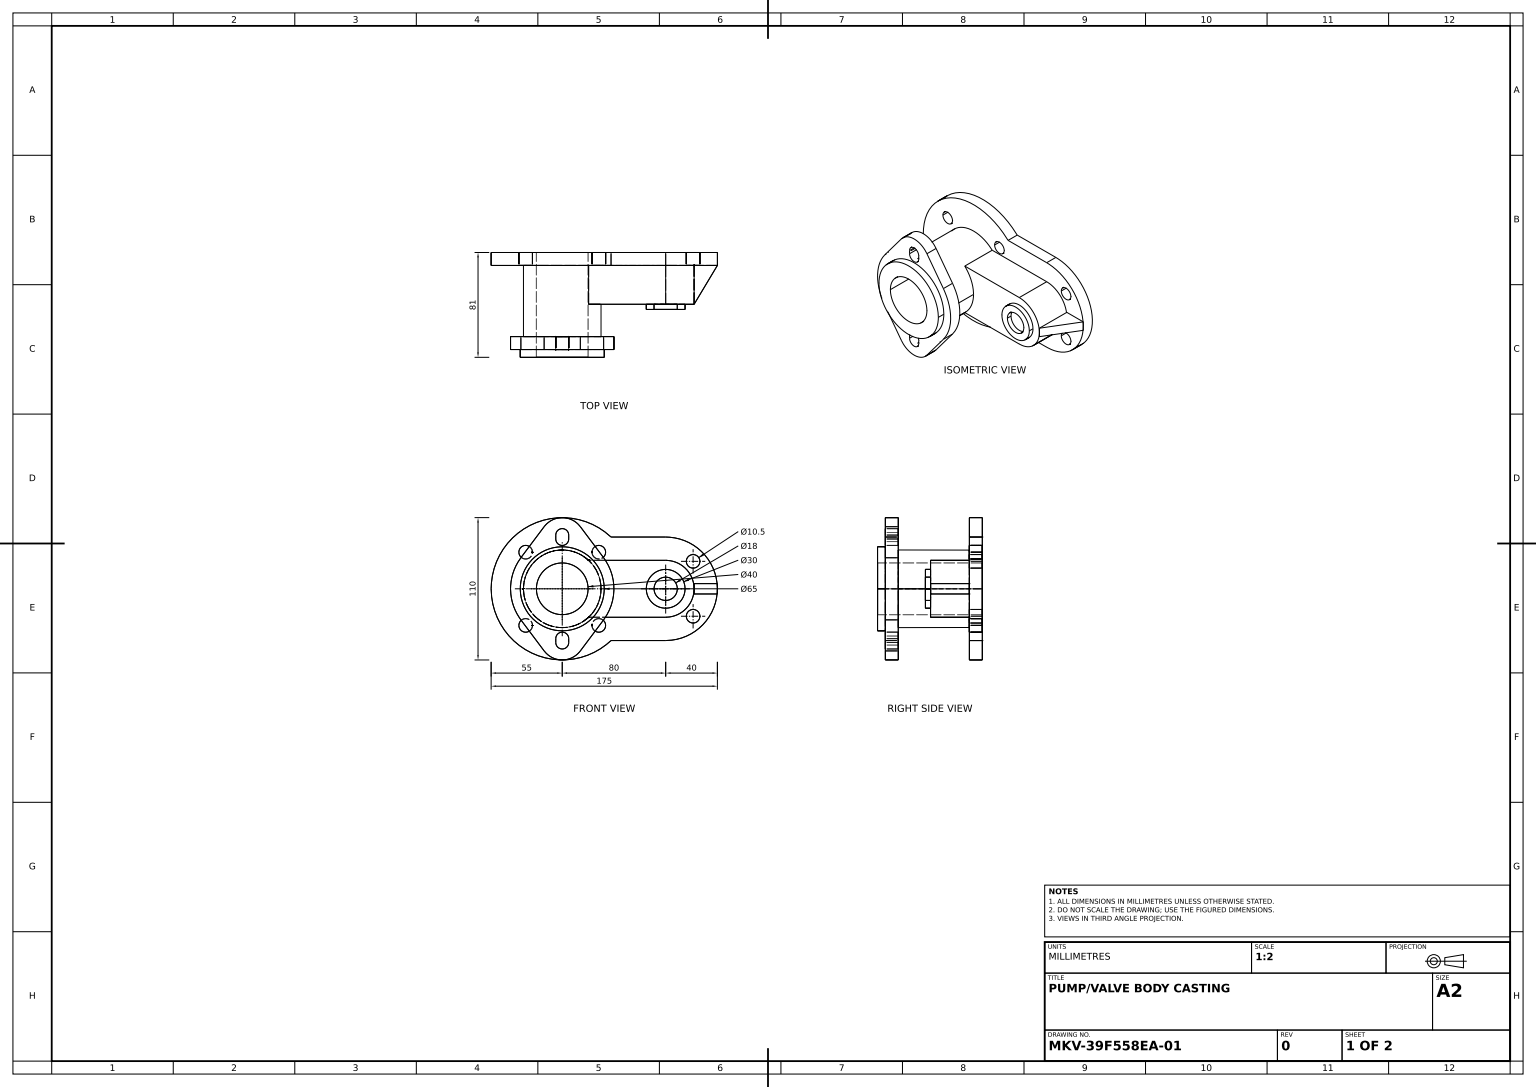
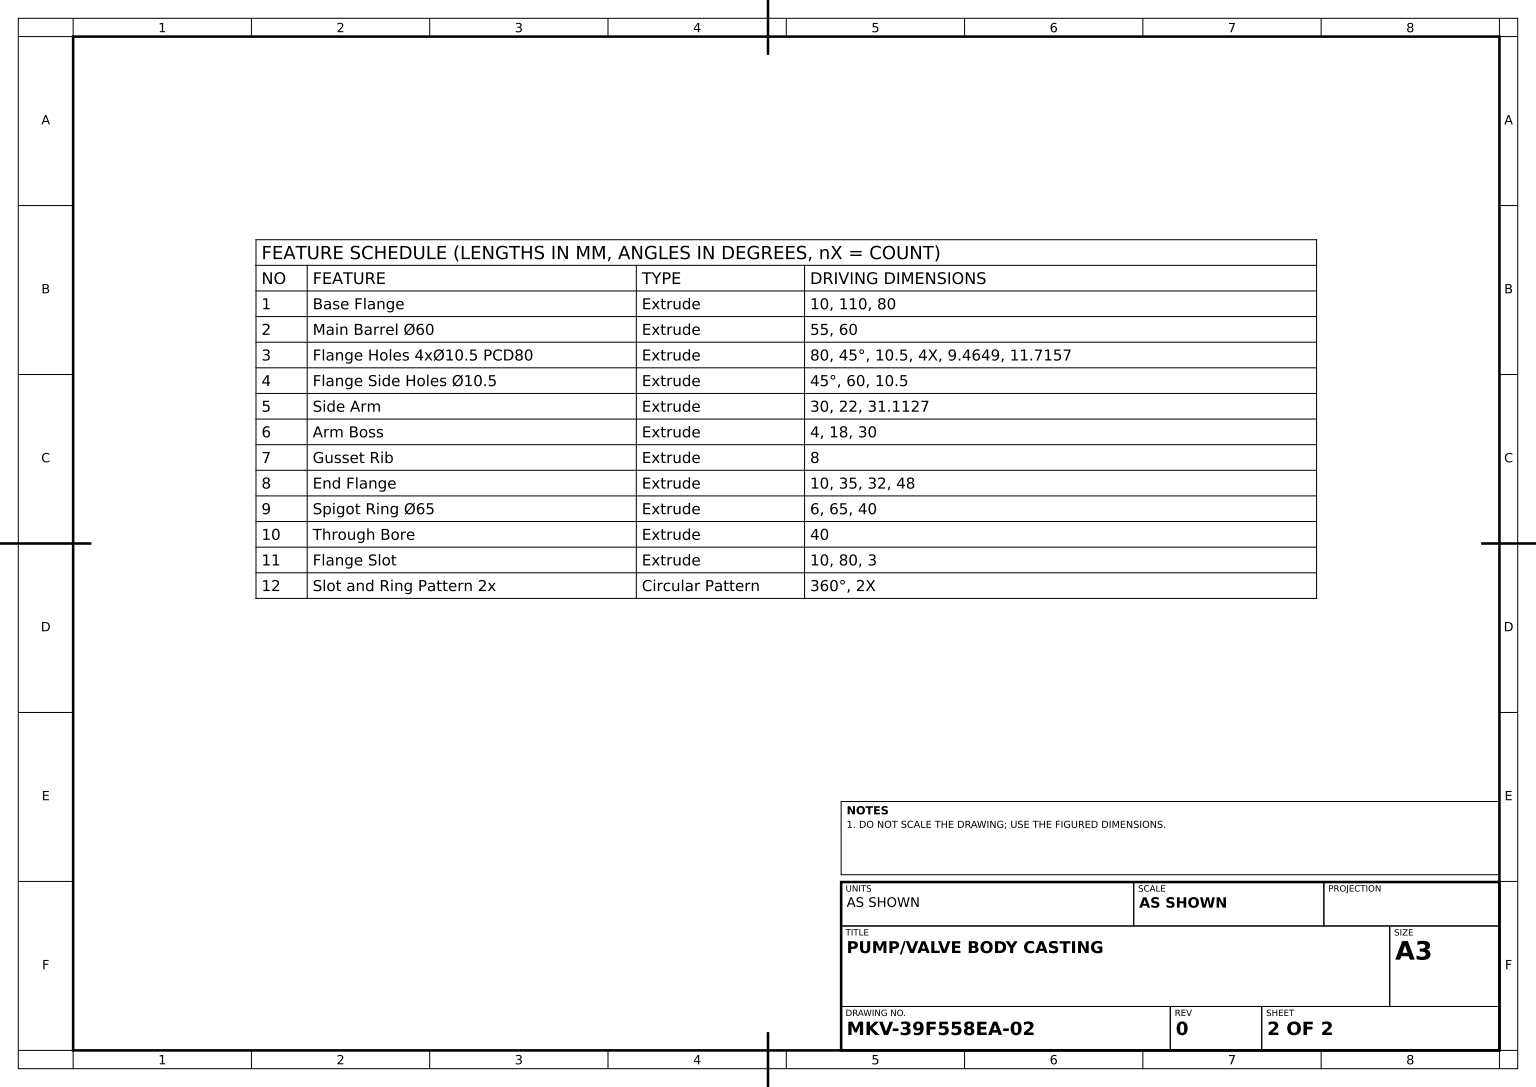
solid
v1 (102,4,40)
v2 (102,-4,40)
e1 v1 v2 LINE
v3 (102,4,10)
e2 v3 v1 LINE
v4 (102,-4,10)
e3 v3 v4 LINE
e4 v4 v2 LINE
face PLANE(AX(P(102,4,40),D(1,0,0),D(0,0,-1))) rev [-e1 -e2 e3 e4]
v5 (120,-4,10)
e5 v5 v4 LINE
v6 (120,4,10)
e6 v6 v3 LINE
e7 v6 v5 LINE
face PLANE(AX(P(102,4,10),D(0,0,1),D(1,0,0))) rev [e5 -e3 -e6 e7]
e8 v1 v6 LINE
face PLANE(AX(P(0,4,0),D(0,-1,0),D(0,0,-1))) rev [e6 e2 e8]
e9 v2 v5 LINE
face PLANE(AX(P(0,-4,0),D(0,-1,0),D(0,0,-1))) [-e4 -e5 -e9]
face PLANE(AX(P(102,4,40),D(-0.857492926,0,-0.514495755),D(-0.514495755,0,0.857492926))) rev [-e8 e1 e9 -e7]
solid
v7 (-5,41.5,65)
v8 (-5,41.5,75)
e10 v7 v8 LINE
v9 (5,41.5,65)
e11 v9 v7 CIRCLE(AX(P(0,41.5,65),D(0,0,1),D(1,0,0)),5)
v10 (5,41.5,75)
e12 v9 v10 LINE
e13 v10 v8 CIRCLE(AX(P(0,41.5,75),D(0,0,1),D(1,0,0)),5)
face CYL(AX(P(0,41.5,65),D(0,0,1),D(1,0,0)),5) rev [-e10 -e11 e12 e13]
v11 (80,-40,10)
v12 (80,-40,0)
e14 v11 v12 LINE
v13 (37.749172,-40,10)
e15 v13 v11 LINE
v14 (37.749172,-40,0)
e16 v13 v14 LINE
e17 v14 v12 LINE
face PLANE(AX(P(80,-40,10),D(0,1,0),D(0,0,1))) rev [-e14 -e15 e16 e17]
v15 (30,0,65)
v16 (-30,0,65)
e18 v15 v16 CIRCLE(AX(P(0,0,65),D(0,0,1),D(1,0,0)),30)
v17 (30,0,40)
e19 v15 v17 LINE
v18 (20.396078,22,40)
e20 v17 v18 CIRCLE(AX(P(0,0,40),D(0,0,1),D(1,0,0)),30)
v19 (20.396078,22,10)
e21 v18 v19 LINE
v20 (-30,0,10)
e22 v19 v20 CIRCLE(AX(P(0,0,10),D(0,0,1),D(1,0,0)),30)
e23 v16 v20 LINE
face CYL(AX(P(0,0,65),D(0,0,-1),D(-1,0,0)),30) [-e18 e19 e20 e21 e22 -e23]
v21 (-23.034271,-28.284271,10)
v22 (-33.534271,-28.284271,10)
e24 v21 v22 CIRCLE(AX(P(-28.284271,-28.284271,10),D(0,0,1),D(1,0,0)),5.25)
v23 (-33.534271,-28.284271,0)
e25 v23 v22 LINE
v24 (-23.034271,-28.284271,0)
e26 v24 v23 CIRCLE(AX(P(-28.284271,-28.284271,0),D(0,0,1),D(1,0,0)),5.25)
e27 v24 v21 LINE
face CYL(AX(P(-28.284271,-28.284271,0),D(0,0,1),D(1,0,0)),5.25) rev [e24 -e25 -e26 e27]
v25 (33.534271,-28.284271,0)
v26 (23.034271,-28.284271,0)
e28 v25 v26 CIRCLE(AX(P(28.284271,-28.284271,0),D(0,0,1),D(1,0,0)),5.25)
v27 (33.534271,-28.284271,10)
e29 v25 v27 LINE
v28 (23.034271,-28.284271,10)
e30 v27 v28 CIRCLE(AX(P(28.284271,-28.284271,10),D(0,0,1),D(1,0,0)),5.25)
e31 v26 v28 LINE
face CYL(AX(P(28.284271,-28.284271,0),D(0,0,1),D(1,0,0)),5.25) rev [-e28 e29 e30 -e31]
v29 (65,0,44)
v30 (65,0,40)
e32 v29 v30 LINE
v31 (95,0,40)
e33 v30 v31 CIRCLE(AX(P(80,0,40),D(0,0,1),D(1,0,0)),15)
v32 (95,0,44)
e34 v32 v31 LINE
e35 v29 v32 CIRCLE(AX(P(80,0,44),D(0,0,1),D(1,0,0)),15)
face CYL(AX(P(80,0,44),D(0,0,-1),D(-1,0,0)),15) [e32 e33 -e34 -e35]
v33 (-33.534271,28.284271,10)
v34 (-23.034271,28.284271,10)
e36 v33 v34 CIRCLE(AX(P(-28.284271,28.284271,10),D(0,0,1),D(1,0,0)),5.25)
v35 (-23.034271,28.284271,0)
e37 v35 v34 LINE
v36 (-33.534271,28.284271,0)
e38 v36 v35 CIRCLE(AX(P(-28.284271,28.284271,0),D(0,0,1),D(1,0,0)),5.25)
e39 v36 v33 LINE
face CYL(AX(P(-28.284271,28.284271,0),D(0,0,1),D(1,0,0)),5.25) rev [e36 -e37 -e38 e39]
v37 (106.463203,21.213203,0)
v38 (95.963203,21.213203,0)
e40 v37 v38 CIRCLE(AX(P(101.213203,21.213203,0),D(0,0,1),D(1,0,0)),5.25)
v39 (106.463203,21.213203,10)
e41 v37 v39 LINE
v40 (95.963203,21.213203,10)
e42 v39 v40 CIRCLE(AX(P(101.213203,21.213203,10),D(0,0,1),D(1,0,0)),5.25)
e43 v38 v40 LINE
face CYL(AX(P(101.213203,21.213203,0),D(0,0,1),D(1,0,0)),5.25) rev [-e40 e41 e42 -e43]
v41 (32.5,0,81)
v42 (-32.5,0,81)
e44 v41 v42 CIRCLE(AX(P(0,0,81),D(0,0,1),D(1,0,0)),32.5)
e45 v42 v41 CIRCLE(AX(P(0,0,81),D(0,0,1),D(1,0,0)),32.5)
v43 (-20,0,81)
v44 (20,0,81)
e46 v43 v44 CIRCLE(AX(P(0,0,81),D(0,0,1),D(1,0,0)),20)
e47 v44 v43 CIRCLE(AX(P(0,0,81),D(0,0,1),D(1,0,0)),20)
face PLANE(AX(P(0,0,81),D(0,0,1),D(1,0,0))) [e44 e45] [-e46 -e47]
v45 (106.463203,-21.213203,0)
v46 (95.963203,-21.213203,0)
e48 v45 v46 CIRCLE(AX(P(101.213203,-21.213203,0),D(0,0,1),D(1,0,0)),5.25)
e49 v46 v45 CIRCLE(AX(P(101.213203,-21.213203,0),D(0,0,1),D(1,0,0)),5.25)
v47 (37.749172,40,0)
v48 (-55,0,0)
e50 v47 v48 CIRCLE(AX(P(0,0,0),D(0,0,1),D(1,0,0)),55)
v49 (80,40,0)
e51 v49 v47 LINE
e52 v12 v49 CIRCLE(AX(P(80,0,0),D(0,0,1),D(1,0,0)),40)
e53 v48 v14 CIRCLE(AX(P(0,0,0),D(0,0,1),D(1,0,0)),55)
e54 v35 v36 CIRCLE(AX(P(-28.284271,28.284271,0),D(0,0,1),D(1,0,0)),5.25)
e55 v26 v25 CIRCLE(AX(P(28.284271,-28.284271,0),D(0,0,1),D(1,0,0)),5.25)
v50 (23.034271,28.284271,0)
v51 (33.534271,28.284271,0)
e56 v50 v51 CIRCLE(AX(P(28.284271,28.284271,0),D(0,0,1),D(1,0,0)),5.25)
e57 v51 v50 CIRCLE(AX(P(28.284271,28.284271,0),D(0,0,1),D(1,0,0)),5.25)
v52 (20,0,0)
v53 (-20,0,0)
e58 v52 v53 CIRCLE(AX(P(0,0,0),D(0,0,1),D(1,0,0)),20)
e59 v53 v52 CIRCLE(AX(P(0,0,0),D(0,0,1),D(1,0,0)),20)
e60 v38 v37 CIRCLE(AX(P(101.213203,21.213203,0),D(0,0,1),D(1,0,0)),5.25)
e61 v23 v24 CIRCLE(AX(P(-28.284271,-28.284271,0),D(0,0,1),D(1,0,0)),5.25)
face PLANE(AX(P(80,0,0),D(0,0,1),D(1,0,0))) rev [e48 e49] [-e50 -e51 -e52 -e17 -e53] [e38 e54] [e55 e28] [e56 e57] [e58 e59] [e60 e40] [e26 e61]
v54 (20.396078,-22,10)
v55 (80,-22,10)
e62 v54 v55 LINE
e63 v20 v54 CIRCLE(AX(P(0,0,10),D(0,0,1),D(1,0,0)),30)
v56 (80,22,10)
e64 v56 v19 LINE
e65 v55 v56 CIRCLE(AX(P(80,0,10),D(0,0,1),D(1,0,0)),22)
e66 v34 v33 CIRCLE(AX(P(-28.284271,28.284271,10),D(0,0,1),D(1,0,0)),5.25)
v57 (80,40,10)
v58 (37.749172,40,10)
e67 v57 v58 LINE
v59 (-55,0,10)
e68 v58 v59 CIRCLE(AX(P(0,0,10),D(0,0,1),D(1,0,0)),55)
e69 v59 v13 CIRCLE(AX(P(0,0,10),D(0,0,1),D(1,0,0)),55)
e70 v11 v57 CIRCLE(AX(P(80,0,10),D(0,0,1),D(1,0,0)),40)
e71 v40 v39 CIRCLE(AX(P(101.213203,21.213203,10),D(0,0,1),D(1,0,0)),5.25)
v60 (23.034271,28.284271,10)
v61 (33.534271,28.284271,10)
e72 v60 v61 CIRCLE(AX(P(28.284271,28.284271,10),D(0,0,1),D(1,0,0)),5.25)
e73 v61 v60 CIRCLE(AX(P(28.284271,28.284271,10),D(0,0,1),D(1,0,0)),5.25)
e74 v28 v27 CIRCLE(AX(P(28.284271,-28.284271,10),D(0,0,1),D(1,0,0)),5.25)
e75 v22 v21 CIRCLE(AX(P(-28.284271,-28.284271,10),D(0,0,1),D(1,0,0)),5.25)
v62 (106.463203,-21.213203,10)
v63 (95.963203,-21.213203,10)
e76 v62 v63 CIRCLE(AX(P(101.213203,-21.213203,10),D(0,0,1),D(1,0,0)),5.25)
e77 v63 v62 CIRCLE(AX(P(101.213203,-21.213203,10),D(0,0,1),D(1,0,0)),5.25)
face PLANE(AX(P(80,0,10),D(0,0,1),D(1,0,0))) [-e62 -e63 -e22 -e64 -e65] [-e36 -e66] [e67 e68 e69 e15 e70] [-e42 -e71] [-e72 -e73] [-e30 -e74] [-e24 -e75] [-e76 -e77]
face CYL(AX(P(-28.284271,-28.284271,0),D(0,0,1),D(1,0,0)),5.25) rev [-e27 -e61 e25 e75]
v64 (-32,-24,65)
v65 (-14,-48,65)
e78 v64 v65 LINE
v66 (-14,-48,75)
e79 v66 v65 LINE
v67 (-32,-24,75)
e80 v67 v66 LINE
e81 v67 v64 LINE
face PLANE(AX(P(-14,-48,75),D(0.8,0.6,0),D(-0.6,0.8,0))) rev [e78 -e79 -e80 e81]
face CYL(AX(P(101.213203,21.213203,0),D(0,0,1),D(1,0,0)),5.25) rev [-e41 -e60 e43 e71]
v68 (14,48,65)
v69 (-14,48,65)
e82 v68 v69 CIRCLE(AX(P(0,37.5,65),D(0,0,1),D(1,0,0)),17.5)
v70 (-14,48,75)
e83 v70 v69 LINE
v71 (14,48,75)
e84 v71 v70 CIRCLE(AX(P(0,37.5,75),D(0,0,1),D(1,0,0)),17.5)
e85 v71 v68 LINE
face CYL(AX(P(0,37.5,75),D(0,0,-1),D(-1,0,0)),17.5) [e82 -e83 -e84 e85]
v72 (32,24,75)
v73 (32,24,65)
e86 v72 v73 LINE
e87 v73 v68 LINE
e88 v72 v71 LINE
face PLANE(AX(P(14,48,75),D(-0.8,-0.6,0),D(0.6,-0.8,0))) rev [e86 e87 -e85 -e88]
v74 (-5,38.5,65)
e89 v7 v74 LINE
v75 (-5,38.5,75)
e90 v8 v75 LINE
e91 v74 v75 LINE
face PLANE(AX(P(-5,38.5,65),D(-1,0,0),D(0,-1,0))) rev [-e89 e10 e90 -e91]
v76 (5,-41.5,65)
v77 (5,-41.5,75)
e92 v76 v77 LINE
v78 (-5,-41.5,65)
e93 v78 v76 CIRCLE(AX(P(0,-41.5,65),D(0,0,1),D(-1,0,0)),5)
v79 (-5,-41.5,75)
e94 v78 v79 LINE
e95 v79 v77 CIRCLE(AX(P(0,-41.5,75),D(0,0,1),D(-1,0,0)),5)
face CYL(AX(P(0,-41.5,65),D(0,0,1),D(1,0,0)),5) rev [-e92 -e93 e94 e95]
v80 (-32,24,75)
v81 (-32,24,65)
e96 v80 v81 LINE
v82 (-40,0,65)
e97 v81 v82 CIRCLE(AX(P(0,0,65),D(0,0,1),D(1,0,0)),40)
v83 (-40,0,75)
e98 v83 v82 LINE
e99 v80 v83 CIRCLE(AX(P(0,0,75),D(0,0,1),D(1,0,0)),40)
face CYL(AX(P(0,0,75),D(0,0,-1),D(-1,0,0)),40) [e96 e97 -e98 -e99]
v84 (-32.5,0,75)
e100 v42 v84 LINE
v85 (32.5,0,75)
e101 v84 v85 CIRCLE(AX(P(0,0,75),D(0,0,1),D(1,0,0)),32.5)
e102 v41 v85 LINE
face CYL(AX(P(0,0,81),D(0,0,-1),D(-1,0,0)),32.5) [e100 e101 -e102 -e45]
e103 v32 v29 CIRCLE(AX(P(80,0,44),D(0,0,1),D(1,0,0)),15)
v86 (89,0,44)
v87 (71,0,44)
e104 v86 v87 CIRCLE(AX(P(80,0,44),D(0,0,1),D(1,0,0)),9)
e105 v87 v86 CIRCLE(AX(P(80,0,44),D(0,0,1),D(1,0,0)),9)
face PLANE(AX(P(80,0,44),D(0,0,1),D(1,0,0))) [e35 e103] [-e104 -e105]
v88 (-5,-38.5,75)
e106 v88 v79 LINE
v89 (-5,-38.5,65)
e107 v89 v78 LINE
e108 v89 v88 LINE
face PLANE(AX(P(-5,-38.5,65),D(-1,0,0),D(0,-1,0))) rev [e106 -e94 -e107 e108]
e109 v44 v52 LINE
e110 v43 v53 LINE
face CYL(AX(P(0,0,81),D(0,0,-1),D(-1,0,0)),20) rev [e109 -e59 -e110 e46]
v90 (5,-38.5,75)
e111 v77 v90 LINE
v91 (5,-38.5,65)
e112 v91 v90 LINE
e113 v76 v91 LINE
face PLANE(AX(P(5,-38.5,65),D(1,0,0),D(0,1,0))) rev [e111 -e112 -e113 e92]
v92 (71,0,40)
v93 (89,0,40)
e114 v92 v93 CIRCLE(AX(P(80,0,40),D(0,0,-1),D(1,0,0)),9)
e115 v86 v93 LINE
e116 v87 v92 LINE
face CYL(AX(P(80,0,44),D(0,0,-1),D(-1,0,0)),9) rev [e114 -e115 e104 e116]
face CYL(AX(P(28.284271,-28.284271,0),D(0,0,1),D(1,0,0)),5.25) rev [-e29 -e55 e31 e74]
e117 v93 v92 CIRCLE(AX(P(80,0,40),D(0,0,-1),D(1,0,0)),9)
face PLANE(AX(P(80,0,40),D(0,0,1),D(1,0,0))) [-e117 -e114]
v94 (14,-48,75)
e118 v66 v94 CIRCLE(AX(P(0,-37.5,75),D(0,0,1),D(1,0,0)),17.5)
v95 (14,-48,65)
e119 v65 v95 CIRCLE(AX(P(0,-37.5,65),D(0,0,1),D(1,0,0)),17.5)
e120 v94 v95 LINE
face CYL(AX(P(0,-37.5,75),D(0,0,-1),D(-1,0,0)),17.5) [-e118 e79 e119 -e120]
e121 v51 v61 LINE
e122 v50 v60 LINE
face CYL(AX(P(28.284271,28.284271,0),D(0,0,1),D(1,0,0)),5.25) rev [e72 -e121 -e56 e122]
v96 (5,38.5,65)
e123 v74 v96 CIRCLE(AX(P(0,38.5,65),D(0,0,1),D(1,0,0)),5)
e124 v96 v9 LINE
e125 v16 v15 CIRCLE(AX(P(0,0,65),D(0,0,1),D(1,0,0)),30)
e126 v91 v89 CIRCLE(AX(P(0,-38.5,65),D(0,0,1),D(-1,0,0)),5)
v97 (32,-24,65)
e127 v97 v73 CIRCLE(AX(P(0,0,65),D(0,0,1),D(1,0,0)),40)
e128 v95 v97 LINE
e129 v82 v64 CIRCLE(AX(P(0,0,65),D(0,0,1),D(1,0,0)),40)
e130 v69 v81 LINE
face PLANE(AX(P(0,37.5,65),D(0,0,1),D(1,0,0))) rev [e123 e124 e11 e89] [e18 e125] [e126 e107 e93 e113] [-e87 -e127 -e128 -e119 -e78 -e129 -e97 -e130 -e82]
e131 v59 v48 LINE
e132 v58 v47 LINE
face CYL(AX(P(0,0,10),D(0,0,-1),D(-1,0,0)),55) [-e131 -e68 e132 e50]
v98 (20.396078,-22,40)
e133 v98 v17 CIRCLE(AX(P(0,0,40),D(0,0,1),D(1,0,0)),30)
e134 v98 v54 LINE
face CYL(AX(P(0,0,65),D(0,0,-1),D(-1,0,0)),30) [e133 -e19 -e125 e23 e63 -e134]
v99 (80,22,40)
e135 v99 v18 LINE
e136 v99 v56 LINE
face PLANE(AX(P(80,22,40),D(0,-1,0),D(0,0,-1))) rev [-e21 -e135 e136 e64]
e137 v46 v63 LINE
e138 v45 v62 LINE
face CYL(AX(P(101.213203,-21.213203,0),D(0,0,1),D(1,0,0)),5.25) rev [-e137 -e48 e138 e76]
v100 (5,38.5,75)
e139 v75 v100 CIRCLE(AX(P(0,38.5,75),D(0,0,1),D(1,0,0)),5)
e140 v96 v100 LINE
face CYL(AX(P(0,38.5,65),D(0,0,1),D(1,0,0)),5) rev [e139 -e140 -e123 e91]
e141 v70 v80 LINE
face PLANE(AX(P(-14,48,75),D(0.8,-0.6,0),D(0.6,0.8,0))) rev [e130 -e96 -e141 e83]
e142 v90 v88 CIRCLE(AX(P(0,-38.5,75),D(0,0,1),D(-1,0,0)),5)
face CYL(AX(P(0,-38.5,65),D(0,0,1),D(1,0,0)),5) rev [e112 e142 -e108 -e126]
e143 v83 v67 CIRCLE(AX(P(0,0,75),D(0,0,1),D(1,0,0)),40)
v101 (32,-24,75)
e144 v94 v101 LINE
e145 v101 v72 CIRCLE(AX(P(0,0,75),D(0,0,1),D(1,0,0)),40)
e146 v85 v84 CIRCLE(AX(P(0,0,75),D(0,0,1),D(1,0,0)),32.5)
e147 v100 v10 LINE
face PLANE(AX(P(0,37.5,75),D(0,0,1),D(1,0,0))) [-e142 -e111 -e95 -e106] [e88 e84 e141 e99 e143 e80 e118 e144 e145] [-e146 -e101] [-e90 -e13 -e147 -e139]
face CYL(AX(P(-28.284271,28.284271,0),D(0,0,1),D(1,0,0)),5.25) rev [e66 -e39 -e54 e37]
e148 v57 v49 LINE
face CYL(AX(P(80,0,10),D(0,0,-1),D(-1,0,0)),40) [e52 -e148 -e70 e14]
e149 v101 v97 LINE
face CYL(AX(P(0,0,75),D(0,0,-1),D(-1,0,0)),40) [e127 -e86 -e145 e149]
face CYL(AX(P(80,0,44),D(0,0,-1),D(-1,0,0)),9) rev [-e116 e105 e115 e117]
face PLANE(AX(P(5,38.5,65),D(1,0,0),D(0,1,0))) rev [-e124 e140 e147 -e12]
v102 (80,-22,40)
e150 v98 v102 LINE
e151 v102 v99 CIRCLE(AX(P(80,0,40),D(0,0,1),D(1,0,0)),22)
e152 v31 v30 CIRCLE(AX(P(80,0,40),D(0,0,1),D(1,0,0)),15)
face PLANE(AX(P(80,0,40),D(0,0,1),D(1,0,0))) [e150 e151 e135 -e20 -e133] [-e33 -e152]
face CYL(AX(P(28.284271,28.284271,0),D(0,0,1),D(1,0,0)),5.25) rev [-e122 -e57 e121 e73]
face PLANE(AX(P(14,-48,75),D(-0.8,0.6,0),D(-0.6,-0.8,0))) rev [e120 e128 -e149 -e144]
e153 v102 v55 LINE
face PLANE(AX(P(80,-22,40),D(0,1,0),D(0,0,1))) rev [-e150 e134 e62 -e153]
face CYL(AX(P(0,0,10),D(0,0,-1),D(-1,0,0)),55) [-e69 e131 e53 -e16]
face CYL(AX(P(80,0,44),D(0,0,-1),D(-1,0,0)),15) [-e103 e34 e152 -e32]
face PLANE(AX(P(80,40,10),D(0,-1,0),D(0,0,-1))) rev [e148 e51 -e132 -e67]
face CYL(AX(P(80,0,40),D(0,0,-1),D(-1,0,0)),22) [e65 -e136 -e151 e153]
face CYL(AX(P(0,0,81),D(0,0,-1),D(-1,0,0)),20) rev [e47 e110 -e58 -e109]
face CYL(AX(P(0,0,75),D(0,0,-1),D(-1,0,0)),40) [e98 e129 -e81 -e143]
face CYL(AX(P(0,0,81),D(0,0,-1),D(-1,0,0)),32.5) [-e44 e102 e146 -e100]
face CYL(AX(P(101.213203,-21.213203,0),D(0,0,1),D(1,0,0)),5.25) rev [e137 e77 -e138 -e49]
